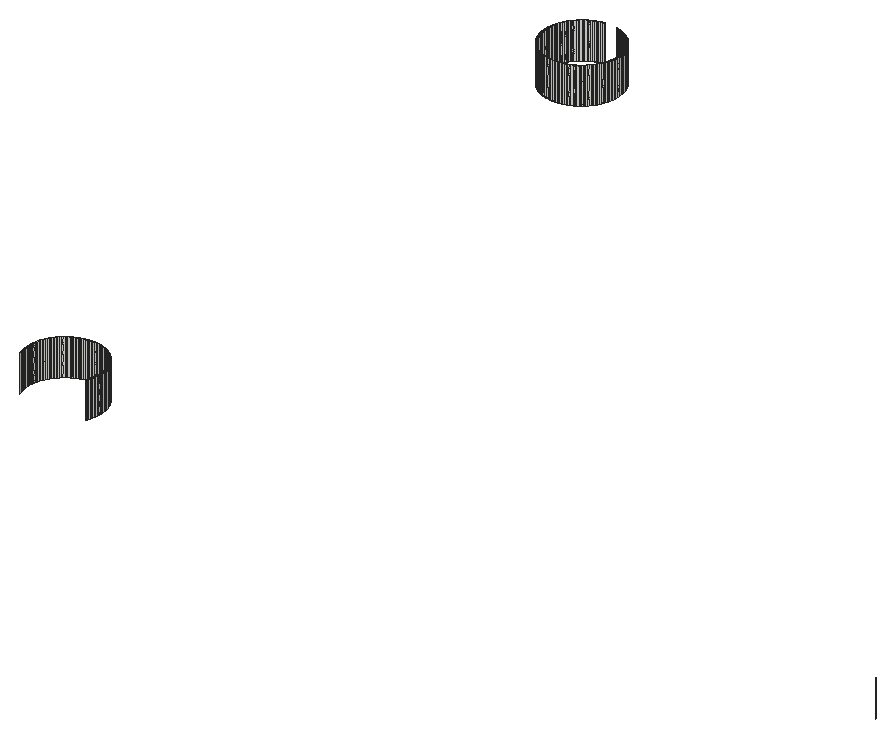
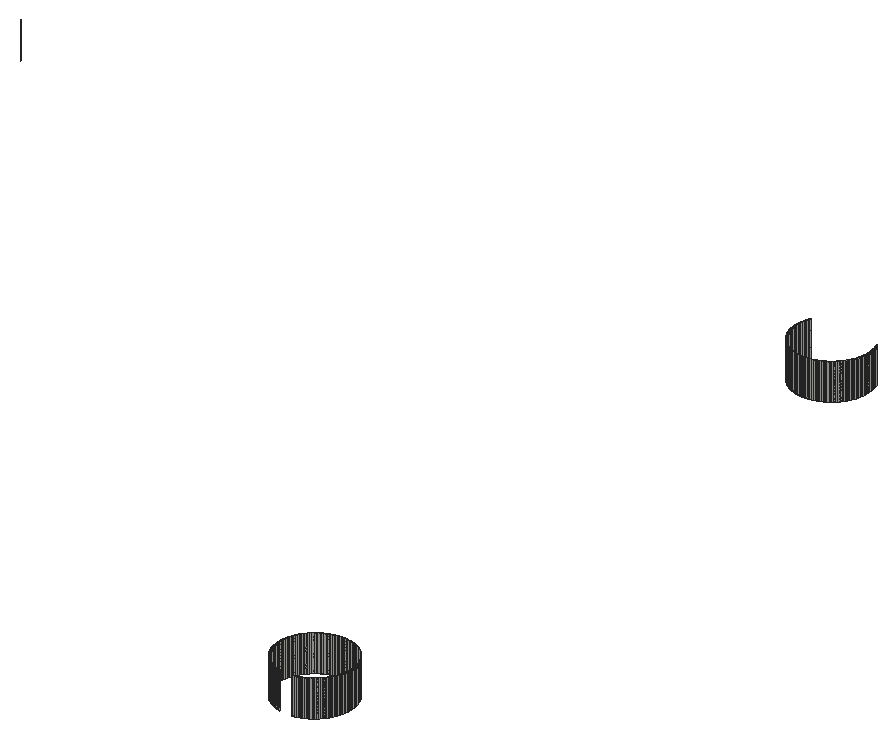
# SketchUp Ruby script. Lengths in inches.
U = 1.inch
M = Sketchup.active_model
def pt(a) = Geom::Point3d.new(a.map { |v| v * U })
def face(e, loops, mat)
  f = e.add_face(loops[0].map { |a| pt(a) })
  loops[1..].each { |l| e.add_face(l.map { |a| pt(a) }).erase! }
  f.material = f.back_material = mat if mat
  f
end
# faces: each face lists its corners as indices into pts; further lists are holes
def faces(e, pts, list, mat = nil) = list.each { |f| face(e, (f[0].is_a?(Array) ? f : [f]).map { |l| l.map { |i| pts[i] } }, mat) }
# xy, xz, yz: faces in a plane at the given z, y or x. An outline is a flat list of corners, or four numbers for a rectangle; further outlines are holes
def ring(l) = l.size == 4 ? [[l[0], l[1]], [l[2], l[1]], [l[2], l[3]], [l[0], l[3]]] : l.each_slice(2).to_a
def flat(e, list, mat, &to3) = list.each { |f| face(e, (f[0].is_a?(Array) ? f : [f]).map { |l| ring(l).map { |u, v| to3.(u, v) } }, mat) }
def xy(e, z, list, mat = nil) = flat(e, list, mat) { |x, y| [x, y, z] }
def xz(e, y, list, mat = nil) = flat(e, list, mat) { |x, z| [x, y, z] }
def yz(e, x, list, mat = nil) = flat(e, list, mat) { |y, z| [x, y, z] }
def lines(e, pts, list) = list.each { |a, b| e.add_line(pt(pts[a]), pt(pts[b])) }
# prism: a flat outline (further loops are holes) pulled along v
def prism(e, loops, v, mat = nil)
  f = face(e, loops, mat); d = Geom::Vector3d.new(v.map { |x| x * U })
  f.pushpull(f.normal.samedirection?(d) ? d.length : -d.length)
end
def box(e, o, s, mat = nil) = prism(e, [[o, [o[0] + s[0], o[1], o[2]], [o[0] + s[0], o[1] + s[1], o[2]], [o[0], o[1] + s[1], o[2]]]], [0, 0, s[2]], mat)
def at(x, y, z, deg = 0) = Geom::Transformation.translation(pt([x, y, z])) * Geom::Transformation.rotation(ORIGIN, Z_AXIS, deg.degrees)
def axes(o, x, y, z) = Geom::Transformation.new([*x, 0, *y, 0, *z, 0, *pt(o).to_a, 1])
def part(name) = M.definitions.add(name)
# library, detail: a bought-in or finely detailed component or shape, given as its bounding box
def library(name, o, s) = part(name).tap { |d| box(d.entities, o, s) }
def detail(e, o, s) = box(e.add_group.entities, o, s)
def put(e, d, t, mat = nil) = e.add_instance(d, t).tap { |i| i.material = mat if mat }
def group(e, t, mat = nil) = e.add_group.tap { |g| g.transformation = t; g.material = mat if mat }.entities
root = M.entities
xz(root,178.75,[[30.34,129,30.42,132],[30.42,129,30.5,132],[30.5,129,30.58,132],[30.58,129,30.66,132]])
xz(root,226.5,[[30.34,129,30.42,132],[30.42,129,30.5,132],[30.5,129,30.58,132],[30.58,129,30.66,132]])
yz(root,27.5,[[175.59,129,175.67,132],[175.67,129,175.75,132],[175.75,129,175.83,132],[175.83,129,175.91,132],[229.34,129,229.42,132],
  [229.42,129,229.5,132],[229.5,129,229.58,132],[229.58,129,229.66,132]])
yz(root,33.5,[[175.59,129,175.67,132],[175.67,129,175.75,132],[175.75,129,175.83,132],[175.83,129,175.91,132],[229.34,129,229.42,132],
  [229.42,129,229.5,132],[229.5,129,229.58,132],[229.58,129,229.66,132]])
yz(root,98,[[175.67,129,175.75,132]])
p = [[33.27,174.6,129],[33.24,174.53,129],[33.24,174.53,132],[33.27,174.6,132],[27.73,174.6,129],[27.7,174.67,129],
  [27.7,174.67,132],[27.73,174.6,132],[33.3,174.67,129],[33.3,174.67,132],[27.67,174.75,129],[27.65,174.82,129],
  [27.65,174.82,132],[27.67,174.75,132],[33.33,174.75,129],[33.33,174.75,132],[33.35,174.82,129],[33.35,174.82,132],
  [27.625,174.9,129],[27.625,174.9,132],[33.375,174.9,129],[33.375,174.9,132],[27.6,174.97,129],[27.6,174.97,132],
  [33.4,174.97,129],[33.4,174.97,132],[27.58,175.05,129],[27.57,175.125,129],[27.57,175.125,132],[27.58,175.05,132],
  [33.42,175.05,129],[33.42,175.05,132],[33.43,175.125,129],[33.43,175.125,132],[27.55,175.2,129],[27.55,175.2,132],
  [33.45,175.2,129],[33.45,175.2,132],[27.54,175.28,129],[27.54,175.28,132],[33.46,175.28,129],[33.46,175.28,132],
  [27.53,175.36,129],[27.53,175.36,132],[33.47,175.36,129],[33.47,175.36,132],[27.52,175.4375,129],[27.51,175.51,129],
  [27.51,175.51,132],[27.52,175.4375,132],[33.48,175.4375,129],[33.48,175.4375,132],[33.49,175.51,129],[33.49,175.51,132],
  [27.5,175.59,129],[27.5,175.59,132],[33.5,175.59,129],[33.5,175.59,132],[27.5,175.91,129],[27.51,175.99,129],
  [27.51,175.99,132],[27.5,175.91,132],[33.49,175.99,129],[33.5,175.91,129],[33.5,175.91,132],[33.49,175.99,132],
  [27.52,176.0625,129],[27.52,176.0625,132],[33.48,176.0625,129],[33.48,176.0625,132],[27.53,176.14,129],[27.53,176.14,132],
  [27.54,176.22,129],[27.54,176.22,132],[33.46,176.22,129],[33.47,176.14,129],[33.47,176.14,132],[33.46,176.22,132],
  [27.55,176.3,129],[27.55,176.3,132],[33.45,176.3,129],[33.45,176.3,132],[27.57,176.375,129],[27.57,176.375,132],
  [33.43,176.375,129],[33.43,176.375,132],[27.58,176.45,129],[27.58,176.45,132],[33.42,176.45,129],[33.42,176.45,132],
  [27.6,176.53,129],[27.6,176.53,132],[27.625,176.6,129],[27.625,176.6,132],[33.375,176.6,129],[33.4,176.53,129],
  [33.4,176.53,132],[33.375,176.6,132],[27.65,176.68,129],[27.65,176.68,132],[33.35,176.68,129],[33.35,176.68,132],
  [27.67,176.75,129],[27.67,176.75,132],[33.33,176.75,129],[33.33,176.75,132],[27.7,176.83,129],[27.7,176.83,132],
  [27.73,176.9,129],[27.73,176.9,132],[33.27,176.9,129],[33.3,176.83,129],[33.3,176.83,132],[33.27,176.9,132],
  [27.76,176.97,129],[27.76,176.97,132],[33.24,176.97,129],[33.24,176.97,132],[27.79,177.04,129],[27.79,177.04,132],
  [27.83,177.11,129],[27.83,177.11,132],[33.17,177.11,129],[33.21,177.04,129],[33.21,177.04,132],[33.17,177.11,132],
  [27.86,177.18,129],[27.86,177.18,132],[33.14,177.18,129],[33.14,177.18,132],[27.9,177.25,129],[27.9,177.25,132],
  [27.94,177.32,129],[27.94,177.32,132],[33.06,177.32,129],[33.1,177.25,129],[33.1,177.25,132],[33.06,177.32,132],
  [27.98,177.38,129],[27.98,177.38,132],[33.02,177.38,129],[33.02,177.38,132],[28.03,177.45,129],[28.03,177.45,132],
  [28.07,177.51,129],[28.07,177.51,132],[32.93,177.51,129],[32.97,177.45,129],[32.97,177.45,132],[32.93,177.51,132],
  [28.12,177.58,129],[28.12,177.58,132],[32.88,177.58,129],[32.88,177.58,132],[28.17,177.64,129],[28.17,177.64,132],
  [28.22,177.7,129],[28.22,177.7,132],[32.78,177.7,129],[32.83,177.64,129],[32.83,177.64,132],[32.78,177.7,132],
  [28.27,177.76,129],[28.27,177.76,132],[32.73,177.76,129],[32.73,177.76,132],[28.32,177.82,129],[28.32,177.82,132],
  [28.38,177.87,129],[28.38,177.87,132],[32.62,177.87,129],[32.68,177.82,129],[32.68,177.82,132],[32.62,177.87,132],
  [28.43,177.93,129],[28.43,177.93,132],[28.49,177.98,129],[28.49,177.98,132],[32.51,177.98,129],[32.57,177.93,129],
  [32.57,177.93,132],[32.51,177.98,132],[28.55,178.03,129],[28.55,178.03,132],[28.61,178.08,129],[28.61,178.08,132],
  [32.39,178.08,129],[32.45,178.03,129],[32.45,178.03,132],[32.39,178.08,132],[28.67,178.13,129],[28.67,178.13,132],
  [28.74,178.18,129],[28.74,178.18,132],[32.26,178.18,129],[32.33,178.13,129],[32.33,178.13,132],[32.26,178.18,132],
  [28.8,178.22,129],[28.8,178.22,132],[28.87,178.27,129],[28.87,178.27,132],[32.13,178.27,129],[32.2,178.22,129],
  [32.2,178.22,132],[32.13,178.27,132],[28.93,178.31,129],[28.93,178.31,132],[29,178.35,129],[29,178.35,132],
  [29.07,178.39,129],[29.07,178.39,132],[31.93,178.39,129],[32,178.35,129],[32,178.35,132],[31.93,178.39,132],
  [32.07,178.31,129],[32.07,178.31,132],[29.14,178.42,129],[29.14,178.42,132],[29.21,178.46,129],[29.21,178.46,132],
  [31.79,178.46,129],[31.86,178.42,129],[31.86,178.42,132],[31.79,178.46,132],[29.28,178.49,129],[29.28,178.49,132],
  [29.35,178.52,129],[29.35,178.52,132],[29.42,178.55,129],[29.42,178.55,132],[31.58,178.55,129],[31.65,178.52,129],
  [31.65,178.52,132],[31.58,178.55,132],[31.72,178.49,129],[31.72,178.49,132],[29.5,178.58,129],[29.5,178.58,132],
  [29.57,178.6,129],[29.57,178.6,132],[29.65,178.625,129],[29.65,178.625,132],[29.72,178.65,129],[29.72,178.65,132],
  [29.8,178.67,129],[29.8,178.67,132],[31.2,178.67,129],[31.28,178.65,129],[31.28,178.65,132],[31.2,178.67,132],
  [31.35,178.625,129],[31.35,178.625,132],[31.43,178.6,129],[31.43,178.6,132],[31.5,178.58,129],[31.5,178.58,132],
  [29.875,178.68,129],[29.875,178.68,132],[29.95,178.7,129],[29.95,178.7,132],[30.03,178.71,129],[30.03,178.71,132],
  [30.11,178.72,129],[30.11,178.72,132],[30.1875,178.73,129],[30.1875,178.73,132],[30.26,178.74,129],[30.26,178.74,132],
  [30.34,178.75,129],[30.34,178.75,132],[30.66,178.75,129],[30.74,178.74,129],[30.74,178.74,132],[30.66,178.75,132],
  [30.8125,178.73,129],[30.8125,178.73,132],[30.89,178.72,129],[30.89,178.72,132],[30.97,178.71,129],[30.97,178.71,132],
  [31.05,178.7,129],[31.05,178.7,132],[31.125,178.68,129],[31.125,178.68,132],[30.03,226.54,129],[29.95,226.55,129],
  [29.95,226.55,132],[30.03,226.54,132],[30.11,226.53,129],[30.11,226.53,132],[30.1875,226.52,129],[30.1875,226.52,132],
  [30.26,226.51,129],[30.26,226.51,132],[30.34,226.5,129],[30.34,226.5,132],[30.74,226.51,129],[30.66,226.5,129],
  [30.66,226.5,132],[30.74,226.51,132],[30.8125,226.52,129],[30.8125,226.52,132],[30.89,226.53,129],[30.89,226.53,132],
  [30.97,226.54,129],[30.97,226.54,132],[31.05,226.55,129],[31.05,226.55,132],[29.57,226.65,129],[29.5,226.67,129],
  [29.5,226.67,132],[29.57,226.65,132],[29.65,226.625,129],[29.65,226.625,132],[29.72,226.6,129],[29.72,226.6,132],
  [29.8,226.58,129],[29.8,226.58,132],[29.875,226.57,129],[29.875,226.57,132],[31.125,226.57,129],[31.125,226.57,132],
  [31.2,226.58,129],[31.2,226.58,132],[31.28,226.6,129],[31.28,226.6,132],[31.35,226.625,129],[31.35,226.625,132],
  [31.43,226.65,129],[31.43,226.65,132],[31.5,226.67,129],[31.5,226.67,132],[29.35,226.73,129],[29.28,226.76,129],
  [29.28,226.76,132],[29.35,226.73,132],[29.42,226.7,129],[29.42,226.7,132],[31.58,226.7,129],[31.58,226.7,132],
  [31.65,226.73,129],[31.65,226.73,132],[31.72,226.76,129],[31.72,226.76,132],[29.14,226.83,129],[29.07,226.86,129],
  [29.07,226.86,132],[29.14,226.83,132],[29.21,226.79,129],[29.21,226.79,132],[31.79,226.79,129],[31.79,226.79,132],
  [31.86,226.83,129],[31.86,226.83,132],[31.93,226.86,129],[31.93,226.86,132],[28.93,226.94,129],[28.87,226.98,129],
  [28.87,226.98,132],[28.93,226.94,132],[29,226.9,129],[29,226.9,132],[32,226.9,129],[32,226.9,132],
  [32.07,226.94,129],[32.07,226.94,132],[32.13,226.98,129],[32.13,226.98,132],[28.8,227.03,129],[28.74,227.07,129],
  [28.74,227.07,132],[28.8,227.03,132],[32.2,227.03,129],[32.2,227.03,132],[32.26,227.07,129],[32.26,227.07,132],
  [28.67,227.12,129],[28.61,227.17,129],[28.61,227.17,132],[28.67,227.12,132],[32.33,227.12,129],[32.33,227.12,132],
  [32.39,227.17,129],[32.39,227.17,132],[28.55,227.22,129],[28.49,227.27,129],[28.49,227.27,132],[28.55,227.22,132],
  [32.45,227.22,129],[32.45,227.22,132],[32.51,227.27,129],[32.51,227.27,132],[28.43,227.32,129],[28.38,227.38,129],
  [28.38,227.38,132],[28.43,227.32,132],[32.57,227.32,129],[32.57,227.32,132],[32.62,227.38,129],[32.62,227.38,132],
  [28.32,227.43,129],[28.27,227.49,129],[28.27,227.49,132],[28.32,227.43,132],[32.68,227.43,129],[32.68,227.43,132],
  [32.73,227.49,129],[32.73,227.49,132],[28.22,227.55,129],[28.22,227.55,132],[32.78,227.55,129],[32.78,227.55,132],
  [28.17,227.61,129],[28.12,227.67,129],[28.12,227.67,132],[28.17,227.61,132],[32.83,227.61,129],[32.83,227.61,132],
  [32.88,227.67,129],[32.88,227.67,132],[28.07,227.74,129],[28.03,227.8,129],[28.03,227.8,132],[28.07,227.74,132],
  [32.93,227.74,129],[32.93,227.74,132],[32.97,227.8,129],[32.97,227.8,132],[27.98,227.87,129],[27.98,227.87,132],
  [33.02,227.87,129],[33.02,227.87,132],[27.94,227.93,129],[27.9,228,129],[27.9,228,132],[27.94,227.93,132],
  [33.06,227.93,129],[33.06,227.93,132],[33.1,228,129],[33.1,228,132],[27.86,228.07,129],[27.86,228.07,132],
  [33.14,228.07,129],[33.14,228.07,132],[27.83,228.14,129],[27.79,228.21,129],[27.79,228.21,132],[27.83,228.14,132],
  [33.17,228.14,129],[33.17,228.14,132],[33.21,228.21,129],[33.21,228.21,132],[27.76,228.28,129],[27.76,228.28,132],
  [33.24,228.28,129],[33.24,228.28,132],[27.73,228.35,129],[27.73,228.35,132],[33.27,228.35,129],[33.27,228.35,132],
  [27.7,228.42,129],[27.67,228.5,129],[27.67,228.5,132],[27.7,228.42,132],[33.3,228.42,129],[33.3,228.42,132],
  [33.33,228.5,129],[33.33,228.5,132],[27.65,228.57,129],[27.65,228.57,132],[33.35,228.57,129],[33.35,228.57,132],
  [27.625,228.65,129],[27.6,228.72,129],[27.6,228.72,132],[27.625,228.65,132],[33.375,228.65,129],[33.375,228.65,132],
  [33.4,228.72,129],[33.4,228.72,132],[27.58,228.8,129],[27.58,228.8,132],[33.42,228.8,129],[33.42,228.8,132],
  [27.57,228.875,129],[27.57,228.875,132],[33.43,228.875,129],[33.43,228.875,132],[27.55,228.95,129],[27.55,228.95,132],
  [33.45,228.95,129],[33.45,228.95,132],[27.54,229.03,129],[27.53,229.11,129],[27.53,229.11,132],[27.54,229.03,132],
  [33.46,229.03,129],[33.46,229.03,132],[33.47,229.11,129],[33.47,229.11,132],[27.52,229.1875,129],[27.52,229.1875,132],
  [33.48,229.1875,129],[33.48,229.1875,132],[27.51,229.26,129],[27.51,229.26,132],[33.49,229.26,129],[33.49,229.26,132],
  [27.5,229.34,129],[27.5,229.34,132],[33.5,229.34,129],[33.5,229.34,132],[27.5,229.66,129],[27.51,229.74,129],
  [27.51,229.74,132],[27.5,229.66,132],[27.52,229.8125,129],[27.52,229.8125,132],[33.48,229.8125,129],[33.49,229.74,129],
  [33.49,229.74,132],[33.48,229.8125,132],[33.5,229.66,129],[33.5,229.66,132],[27.53,229.89,129],[27.53,229.89,132],
  [33.47,229.89,129],[33.47,229.89,132],[27.54,229.97,129],[27.54,229.97,132],[33.46,229.97,129],[33.46,229.97,132],
  [27.55,230.05,129],[27.55,230.05,132],[27.57,230.125,129],[27.57,230.125,132],[33.43,230.125,129],[33.45,230.05,129],
  [33.45,230.05,132],[33.43,230.125,132],[27.58,230.2,129],[27.58,230.2,132],[33.42,230.2,129],[33.42,230.2,132],
  [27.6,230.28,129],[27.6,230.28,132],[33.4,230.28,129],[33.4,230.28,132],[27.625,230.35,129],[27.625,230.35,132],
  [33.375,230.35,129],[33.375,230.35,132],[27.65,230.43,129],[27.65,230.43,132],[27.67,230.5,129],[27.67,230.5,132],
  [33.33,230.5,129],[33.35,230.43,129],[33.35,230.43,132],[33.33,230.5,132],[27.7,230.58,129],[27.7,230.58,132],
  [33.3,230.58,129],[33.3,230.58,132],[27.73,230.65,129],[27.73,230.65,132],[27.76,230.72,129],[27.76,230.72,132],
  [33.24,230.72,129],[33.27,230.65,129],[33.27,230.65,132],[33.24,230.72,132],[27.79,230.79,129],[27.79,230.79,132],
  [33.21,230.79,129],[33.21,230.79,132],[27.83,230.86,129],[27.83,230.86,132],[33.17,230.86,129],[33.17,230.86,132],
  [27.86,230.93,129],[27.86,230.93,132],[27.9,231,129],[27.9,231,132],[33.1,231,129],[33.14,230.93,129],
  [33.14,230.93,132],[33.1,231,132],[27.94,231.07,129],[27.94,231.07,132],[33.06,231.07,129],[33.06,231.07,132],
  [27.98,231.13,129],[27.98,231.13,132],[28.03,231.2,129],[28.03,231.2,132],[32.97,231.2,129],[33.02,231.13,129],
  [33.02,231.13,132],[32.97,231.2,132],[28.07,231.26,129],[28.07,231.26,132],[32.93,231.26,129],[32.93,231.26,132],
  [28.12,231.33,129],[28.12,231.33,132],[28.17,231.39,129],[28.17,231.39,132],[32.83,231.39,129],[32.88,231.33,129],
  [32.88,231.33,132],[32.83,231.39,132],[28.22,231.45,129],[28.22,231.45,132],[28.27,231.51,129],[28.27,231.51,132],
  [32.73,231.51,129],[32.78,231.45,129],[32.78,231.45,132],[32.73,231.51,132],[28.32,231.57,129],[28.32,231.57,132],
  [32.68,231.57,129],[32.68,231.57,132],[28.38,231.62,129],[28.38,231.62,132],[28.43,231.68,129],[28.43,231.68,132],
  [32.57,231.68,129],[32.62,231.62,129],[32.62,231.62,132],[32.57,231.68,132],[28.49,231.73,129],[28.49,231.73,132],
  [28.55,231.78,129],[28.55,231.78,132],[32.45,231.78,129],[32.51,231.73,129],[32.51,231.73,132],[32.45,231.78,132],
  [28.61,231.83,129],[28.61,231.83,132],[28.67,231.88,129],[28.67,231.88,132],[32.33,231.88,129],[32.39,231.83,129],
  [32.39,231.83,132],[32.33,231.88,132],[28.74,231.93,129],[28.74,231.93,132],[28.8,231.97,129],[28.8,231.97,132],
  [32.2,231.97,129],[32.26,231.93,129],[32.26,231.93,132],[32.2,231.97,132],[28.87,232.02,129],[28.87,232.02,132],
  [28.93,232.06,129],[28.93,232.06,132],[32.07,232.06,129],[32.13,232.02,129],[32.13,232.02,132],[32.07,232.06,132],
  [29,232.1,129],[29,232.1,132],[29.07,232.14,129],[29.07,232.14,132],[29.14,232.17,129],[29.14,232.17,132],
  [31.86,232.17,129],[31.93,232.14,129],[31.93,232.14,132],[31.86,232.17,132],[32,232.1,129],[32,232.1,132],
  [29.21,232.21,129],[29.21,232.21,132],[29.28,232.24,129],[29.28,232.24,132],[29.35,232.27,129],[29.35,232.27,132],
  [31.65,232.27,129],[31.72,232.24,129],[31.72,232.24,132],[31.65,232.27,132],[31.79,232.21,129],[31.79,232.21,132],
  [29.42,232.3,129],[29.42,232.3,132],[29.5,232.33,129],[29.5,232.33,132],[29.57,232.35,129],[29.57,232.35,132],
  [31.43,232.35,129],[31.5,232.33,129],[31.5,232.33,132],[31.43,232.35,132],[31.58,232.3,129],[31.58,232.3,132],
  [29.65,232.375,129],[29.65,232.375,132],[29.72,232.4,129],[29.72,232.4,132],[29.8,232.42,129],[29.8,232.42,132],
  [29.875,232.43,129],[29.875,232.43,132],[29.95,232.45,129],[29.95,232.45,132],[30.03,232.46,129],[30.03,232.46,132],
  [31.05,232.45,129],[31.125,232.43,129],[31.125,232.43,132],[31.05,232.45,132],[31.2,232.42,129],[31.2,232.42,132],
  [31.28,232.4,129],[31.28,232.4,132],[31.35,232.375,129],[31.35,232.375,132]]
faces(root,p,[[0,1,2,3],[4,5,6,7],[8,0,3,9],[10,11,12,13],[5,10,13,6],[14,8,9,15],[16,14,15,17],[11,18,19,12],
  [20,16,17,21],[18,22,23,19],[24,20,21,25],[26,27,28,29],[22,26,29,23],[30,24,25,31],[32,30,31,33],[27,34,35,28],
  [36,32,33,37],[34,38,39,35],[40,36,37,41],[38,42,43,39],[44,40,41,45],[46,47,48,49],[42,46,49,43],[50,44,45,51],
  [52,50,51,53],[47,54,55,48],[56,52,53,57],[58,59,60,61],[62,63,64,65],[59,66,67,60],[68,62,65,69],[66,70,71,67],
  [70,72,73,71],[74,75,76,77],[75,68,69,76],[72,78,79,73],[80,74,77,81],[78,82,83,79],[84,80,81,85],[82,86,87,83],
  [88,84,85,89],[86,90,91,87],[90,92,93,91],[94,95,96,97],[95,88,89,96],[92,98,99,93],[100,94,97,101],[98,102,103,99],
  [104,100,101,105],[102,106,107,103],[106,108,109,107],[110,111,112,113],[111,104,105,112],[108,114,115,109],[116,110,113,117],[114,118,119,115],
  [118,120,121,119],[122,123,124,125],[123,116,117,124],[120,126,127,121],[128,122,125,129],[126,130,131,127],[130,132,133,131],[134,135,136,137],
  [135,128,129,136],[132,138,139,133],[140,134,137,141],[138,142,143,139],[142,144,145,143],[146,147,148,149],[147,140,141,148],[144,150,151,145],
  [152,146,149,153],[150,154,155,151],[154,156,157,155],[158,159,160,161],[159,152,153,160],[156,162,163,157],[164,158,161,165],[162,166,167,163],
  [166,168,169,167],[170,171,172,173],[171,164,165,172],[168,174,175,169],[174,176,177,175],[178,179,180,181],[179,170,173,180],[176,182,183,177],
  [182,184,185,183],[186,187,188,189],[187,178,181,188],[184,190,191,185],[190,192,193,191],[194,195,196,197],[195,186,189,196],[192,198,199,193],
  [198,200,201,199],[202,203,204,205],[203,194,197,204],[200,206,207,201],[206,208,209,207],[208,210,211,209],[212,213,214,215],[213,216,217,214],
  [216,202,205,217],[210,218,219,211],[218,220,221,219],[222,223,224,225],[223,212,215,224],[220,226,227,221],[226,228,229,227],[228,230,231,229],
  [232,233,234,235],[233,236,237,234],[236,222,225,237],[230,238,239,231],[238,240,241,239],[240,242,243,241],[242,244,245,243],[244,246,247,245],
  [248,249,250,251],[249,252,253,250],[252,254,255,253],[254,256,257,255],[256,232,235,257],[246,258,259,247],[258,260,261,259],[260,262,263,261],
  [262,264,265,263],[264,266,267,265],[266,268,269,267],[268,270,271,269],[272,273,274,275],[273,276,277,274],[276,278,279,277],[278,280,281,279],
  [280,282,283,281],[282,284,285,283],[284,248,251,285],[286,287,288,289],[290,286,289,291],[292,290,291,293],[294,292,293,295],[296,294,295,297],
  [298,299,300,301],[302,298,301,303],[304,302,303,305],[306,304,305,307],[308,306,307,309],[310,311,312,313],[314,310,313,315],[316,314,315,317],
  [318,316,317,319],[320,318,319,321],[287,320,321,288],[322,308,309,323],[324,322,323,325],[326,324,325,327],[328,326,327,329],[330,328,329,331],
  [332,330,331,333],[334,335,336,337],[338,334,337,339],[311,338,339,312],[340,332,333,341],[342,340,341,343],[344,342,343,345],[346,347,348,349],
  [350,346,349,351],[335,350,351,336],[352,344,345,353],[354,352,353,355],[356,354,355,357],[358,359,360,361],[362,358,361,363],[347,362,363,348],
  [364,356,357,365],[366,364,365,367],[368,366,367,369],[370,371,372,373],[359,370,373,360],[374,368,369,375],[376,374,375,377],[378,379,380,381],
  [371,378,381,372],[382,376,377,383],[384,382,383,385],[386,387,388,389],[379,386,389,380],[390,384,385,391],[392,390,391,393],[394,395,396,397],
  [387,394,397,388],[398,392,393,399],[400,398,399,401],[402,403,404,405],[395,402,405,396],[406,400,401,407],[408,406,407,409],[403,410,411,404],
  [412,408,409,413],[414,415,416,417],[410,414,417,411],[418,412,413,419],[420,418,419,421],[422,423,424,425],[415,422,425,416],[426,420,421,427],
  [428,426,427,429],[423,430,431,424],[432,428,429,433],[434,435,436,437],[430,434,437,431],[438,432,433,439],[440,438,439,441],[435,442,443,436],
  [444,440,441,445],[446,447,448,449],[442,446,449,443],[450,444,445,451],[452,450,451,453],[447,454,455,448],[456,452,453,457],[454,458,459,455],
  [460,456,457,461],[462,463,464,465],[458,462,465,459],[466,460,461,467],[468,466,467,469],[463,470,471,464],[472,468,469,473],[474,475,476,477],
  [470,474,477,471],[478,472,473,479],[480,478,479,481],[475,482,483,476],[484,480,481,485],[482,486,487,483],[488,484,485,489],[486,490,491,487],
  [492,488,489,493],[494,495,496,497],[490,494,497,491],[498,492,493,499],[500,498,499,501],[495,502,503,496],[504,500,501,505],[502,506,507,503],
  [508,504,505,509],[506,510,511,507],[512,508,509,513],[514,515,516,517],[515,518,519,516],[520,521,522,523],[521,524,525,522],[518,526,527,519],
  [528,520,523,529],[526,530,531,527],[532,528,529,533],[530,534,535,531],[534,536,537,535],[538,539,540,541],[539,532,533,540],[536,542,543,537],
  [544,538,541,545],[542,546,547,543],[548,544,545,549],[546,550,551,547],[552,548,549,553],[550,554,555,551],[554,556,557,555],[558,559,560,561],
  [559,552,553,560],[556,562,563,557],[564,558,561,565],[562,566,567,563],[566,568,569,567],[570,571,572,573],[571,564,565,572],[568,574,575,569],
  [576,570,573,577],[574,578,579,575],[580,576,577,581],[578,582,583,579],[582,584,585,583],[586,587,588,589],[587,580,581,588],[584,590,591,585],
  [592,586,589,593],[590,594,595,591],[594,596,597,595],[598,599,600,601],[599,592,593,600],[596,602,603,597],[604,598,601,605],[602,606,607,603],
  [606,608,609,607],[610,611,612,613],[611,604,605,612],[608,614,615,609],[614,616,617,615],[618,619,620,621],[619,610,613,620],[616,622,623,617],
  [624,618,621,625],[622,626,627,623],[626,628,629,627],[630,631,632,633],[631,624,625,632],[628,634,635,629],[634,636,637,635],[638,639,640,641],
  [639,630,633,640],[636,642,643,637],[642,644,645,643],[646,647,648,649],[647,638,641,648],[644,650,651,645],[650,652,653,651],[654,655,656,657],
  [655,646,649,656],[652,658,659,653],[658,660,661,659],[662,663,664,665],[663,654,657,664],[660,666,667,661],[666,668,669,667],[668,670,671,669],
  [672,673,674,675],[673,676,677,674],[676,662,665,677],[670,678,679,671],[678,680,681,679],[680,682,683,681],[684,685,686,687],[685,688,689,686],
  [688,672,675,689],[682,690,691,683],[690,692,693,691],[692,694,695,693],[696,697,698,699],[697,700,701,698],[700,684,687,701],[694,702,703,695],
  [702,704,705,703],[704,706,707,705],[706,708,709,707],[708,710,711,709],[710,712,713,711],[714,715,716,717],[715,718,719,716],[718,720,721,719],
  [720,722,723,721],[722,696,699,723]])
